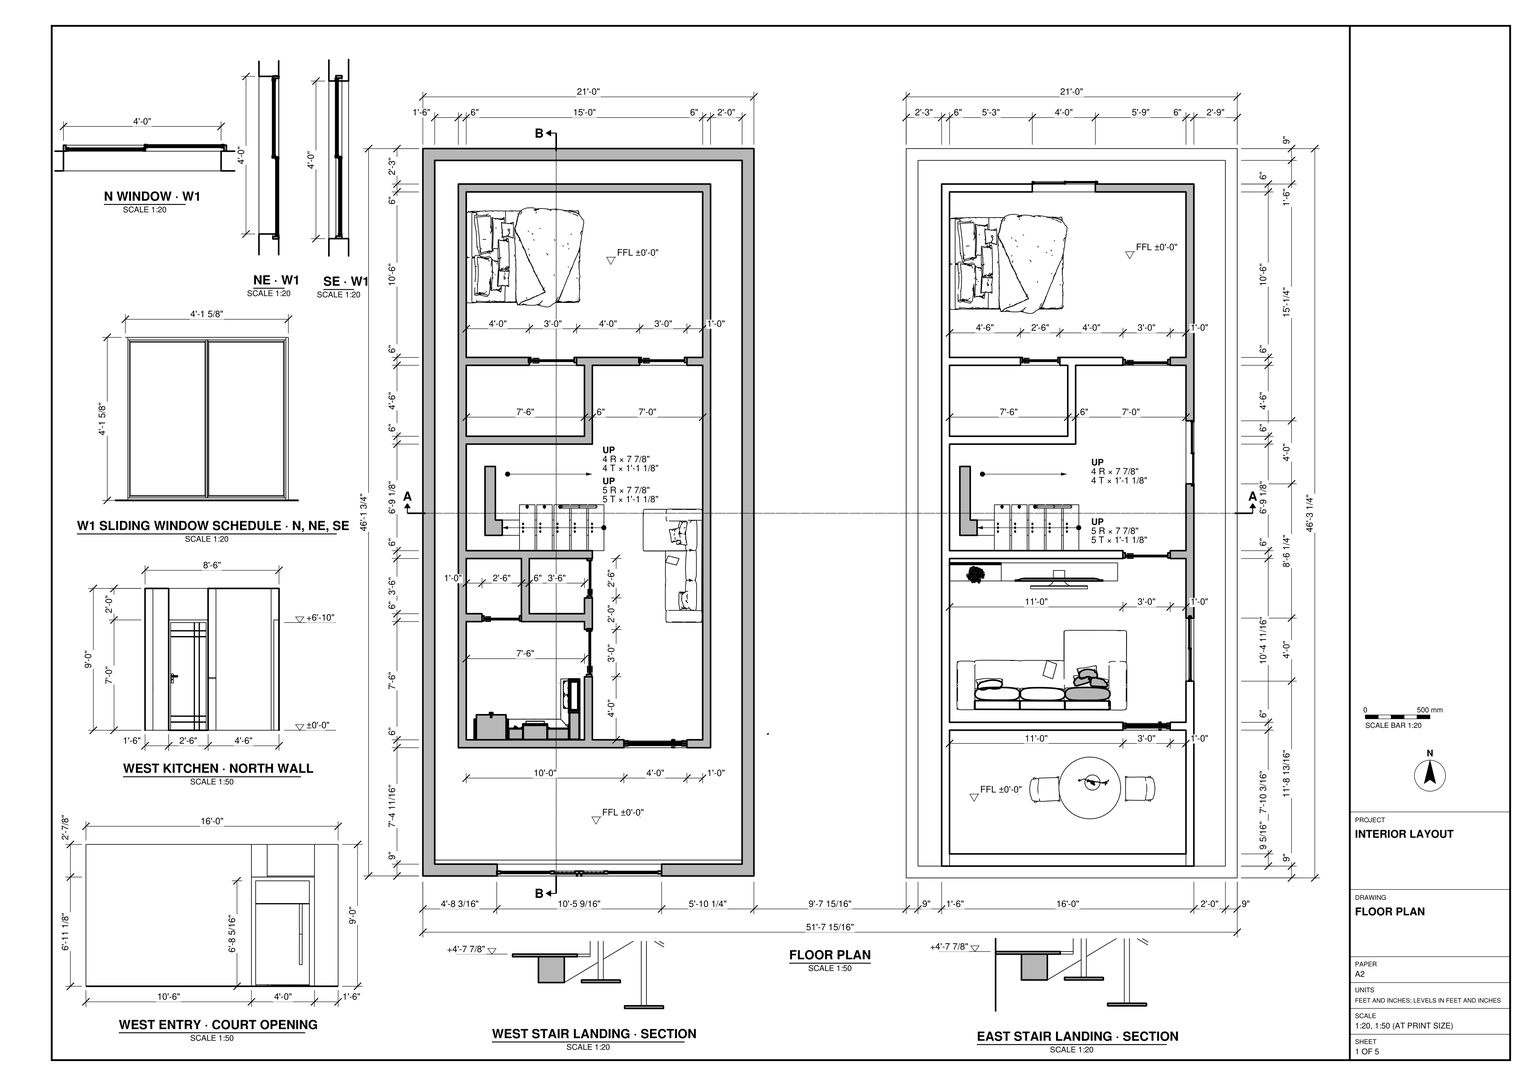
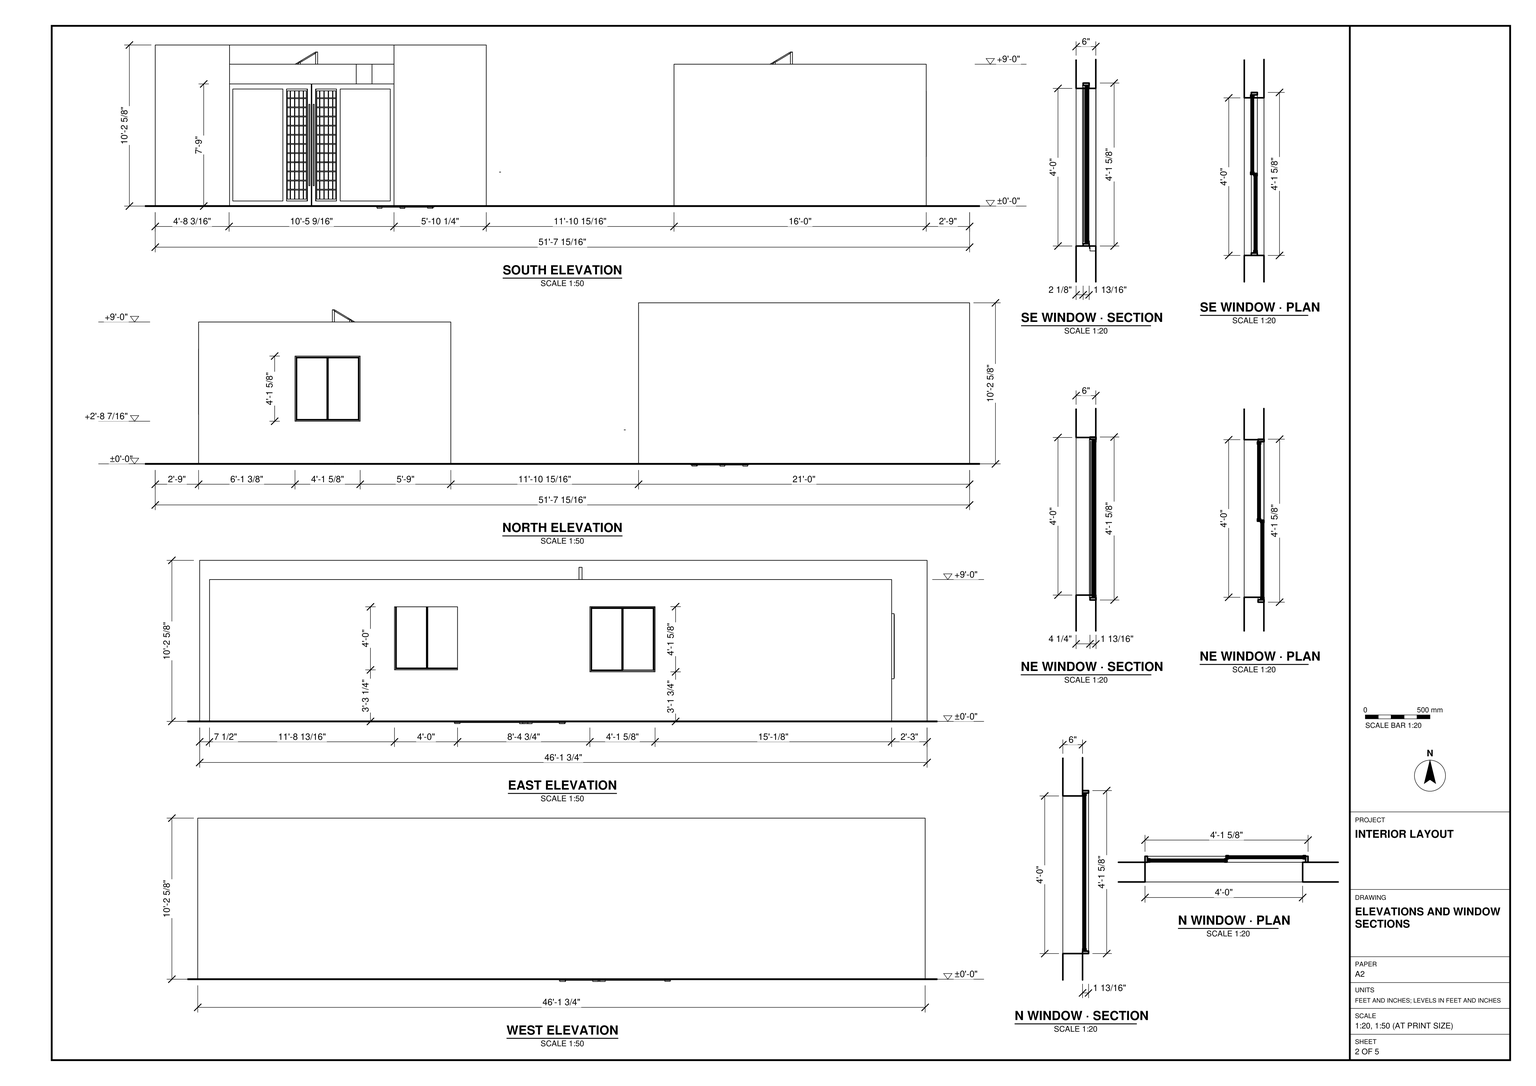
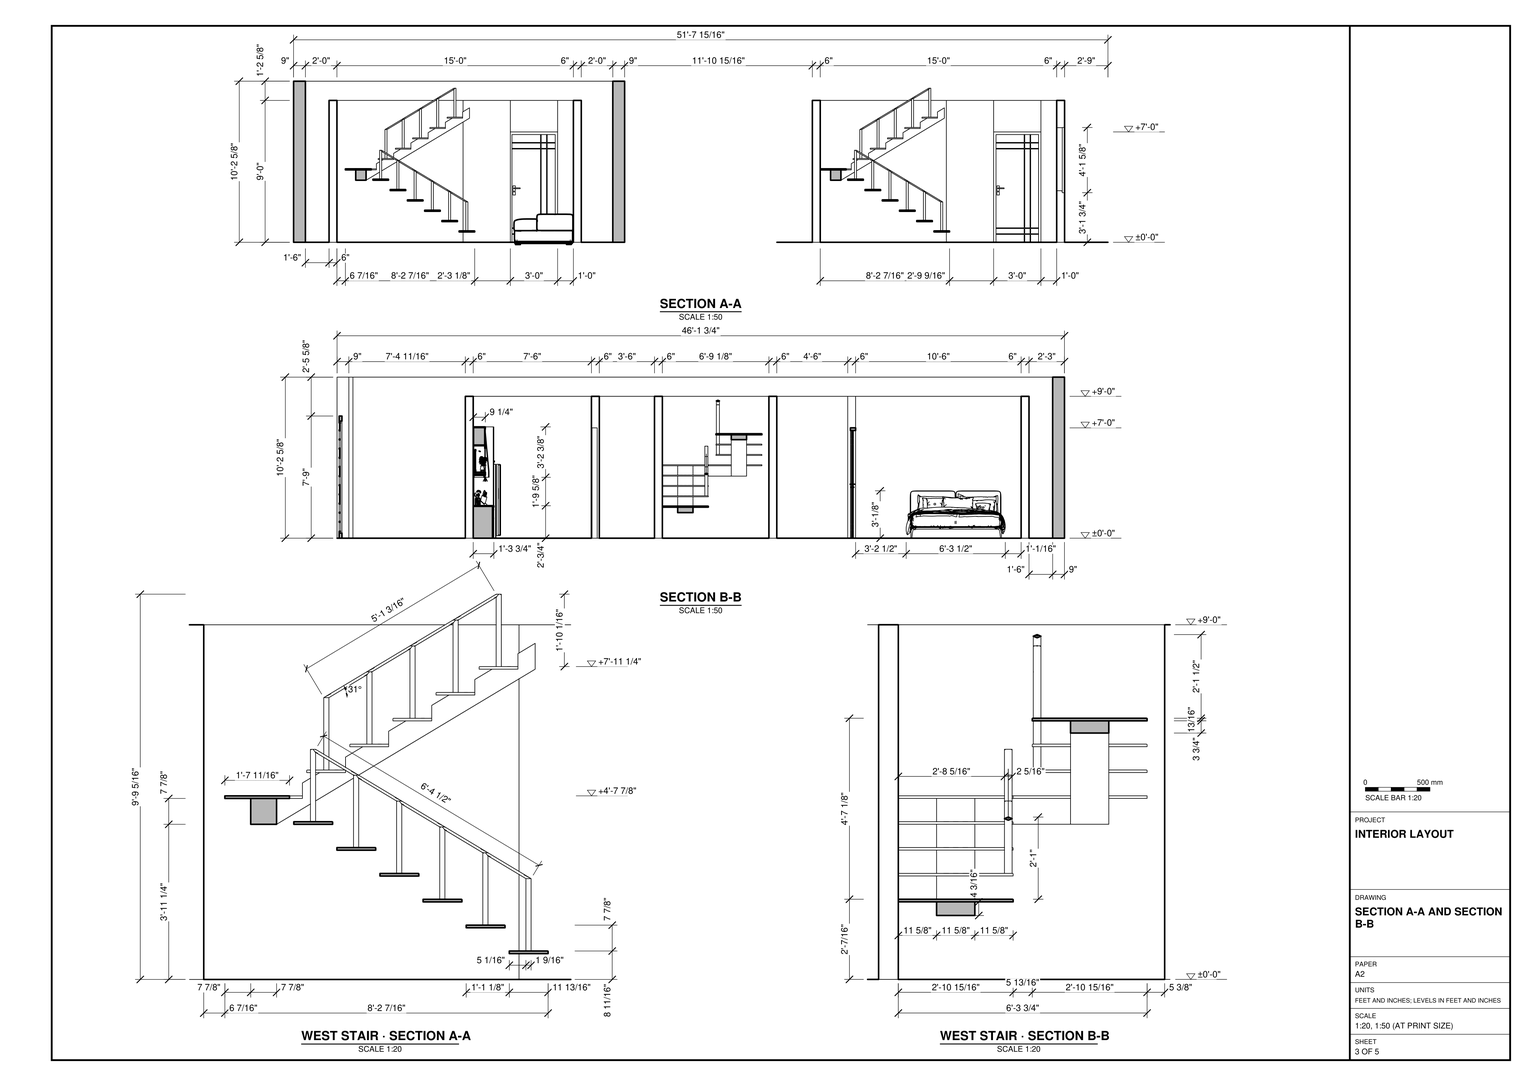
Build both side-by-side layouts in SketchUp from task_files/diagram_01.pdf. Work in feet and inches. Set the finished floor level to ±0'-0" in both layouts. The complete model shall measure 51'-7 15/16" east to west, 46'-3 1/4" north to south and 10'-4 3/8" high. Keep the long axes parallel and use the floor plan to set the gap between the layouts.

Model the floor slabs, the 6" room walls and the taller 9" perimeter walls around the west layout. Form the gated opening into the west entry court and the separate opening from the court into the interior. Place the doors and sliding window units according to the plan, elevations and window details. In the middle of each layout, build the returning stair with individual treads, an intermediate landing, posts and sloping handrails. Use the stair sections to set the heights and the direction in which each flight rises.

Place a bed in each north bedroom. Fit the west kitchen with its L-shaped counter and cabinetry, and place the sofa along the east wall of the west layout. In the east layout, arrange the living room sofa opposite the media unit and furnish the room to its south with the round table and chairs. Match the main furniture and joinery footprints to the plan. Decor, appliances and other loose items may be any suitable library components.

Keep the shell elements and each piece of furniture or joinery in separate groups or components, and use components for repeated parts. Save one SketchUp model as output_files/paired_residential_interiors_and_west_entry_court.skp.

# SketchUp Ruby script. Lengths in inches.
U = 1.inch
M = Sketchup.active_model
def pt(a) = Geom::Point3d.new(a.map { |v| v * U })
def face(e, loops, mat)
  f = e.add_face(loops[0].map { |a| pt(a) })
  loops[1..].each { |l| e.add_face(l.map { |a| pt(a) }).erase! }
  f.material = f.back_material = mat if mat
  f
end
# faces: each face lists its corners as indices into pts; further lists are holes
def faces(e, pts, list, mat = nil) = list.each { |f| face(e, (f[0].is_a?(Array) ? f : [f]).map { |l| l.map { |i| pts[i] } }, mat) }
# xy, xz, yz: faces in a plane at the given z, y or x. An outline is a flat list of corners, or four numbers for a rectangle; further outlines are holes
def ring(l) = l.size == 4 ? [[l[0], l[1]], [l[2], l[1]], [l[2], l[3]], [l[0], l[3]]] : l.each_slice(2).to_a
def flat(e, list, mat, &to3) = list.each { |f| face(e, (f[0].is_a?(Array) ? f : [f]).map { |l| ring(l).map { |u, v| to3.(u, v) } }, mat) }
def xy(e, z, list, mat = nil) = flat(e, list, mat) { |x, y| [x, y, z] }
def xz(e, y, list, mat = nil) = flat(e, list, mat) { |x, z| [x, y, z] }
def yz(e, x, list, mat = nil) = flat(e, list, mat) { |y, z| [x, y, z] }
def lines(e, pts, list) = list.each { |a, b| e.add_line(pt(pts[a]), pt(pts[b])) }
# prism: a flat outline (further loops are holes) pulled along v
def prism(e, loops, v, mat = nil)
  f = face(e, loops, mat); d = Geom::Vector3d.new(v.map { |x| x * U })
  f.pushpull(f.normal.samedirection?(d) ? d.length : -d.length)
end
def box(e, o, s, mat = nil) = prism(e, [[o, [o[0] + s[0], o[1], o[2]], [o[0] + s[0], o[1] + s[1], o[2]], [o[0], o[1] + s[1], o[2]]]], [0, 0, s[2]], mat)
def at(x, y, z, deg = 0) = Geom::Transformation.translation(pt([x, y, z])) * Geom::Transformation.rotation(ORIGIN, Z_AXIS, deg.degrees)
def axes(o, x, y, z) = Geom::Transformation.new([*x, 0, *y, 0, *z, 0, *pt(o).to_a, 1])
def part(name) = M.definitions.add(name)
# library, detail: a bought-in or finely detailed component or shape, given as its bounding box
def library(name, o, s) = part(name).tap { |d| box(d.entities, o, s) }
def detail(e, o, s) = box(e.add_group.entities, o, s)
def put(e, d, t, mat = nil) = e.add_instance(d, t).tap { |i| i.material = mat if mat }
def group(e, t, mat = nil) = e.add_group.tap { |g| g.transformation = t; g.material = mat if mat }.entities
root = M.entities
M.materials.add("Glass_Tinted_Gray").color = [0, 0, 0]
M.materials["Glass_Tinted_Gray"].alpha = 0.125
M.materials.add("[0131_Silver]").color = [192, 192, 192]
M.materials.add("[0135_DarkGray]2").color = [81, 81, 81]
M.materials.add("[Basic Tile]").color = [203, 206, 202]
M.materials.add("[Color M03]").color = [170, 170, 170]
M.materials.add("[Color M05]1").color = [114, 114, 114]
M.materials.add("[Concrete Tile]").color = [203, 190, 164]
M.materials.add("[Field Square Tile]").color = [217, 201, 169]
M.materials.add("[Granite Tile]").color = [155, 148, 143]
M.materials.add("[Grass Dark Green]").color = [106, 157, 55]
M.materials.add("[Metal Panel]").color = [143, 157, 158]
M.materials.add("[Metal_Aluminum_Anodized]").color = [200, 209, 218]
M.materials.add("[Metal_Aluminum_Anodized]1").color = [54, 58, 61]
M.materials.add("[Mirror 02]").color = [229, 229, 229]
M.materials.add("[Quartz Light Brown]").color = [199, 184, 152]
M.materials.add("[Terrazzo Light Blue]").color = [196, 214, 227]
M.materials.add("[Wood Floor]").color = [155, 105, 61]
M.materials.add("[Wood_Board_Cork]").color = [190, 124, 73]
c1 = library("Untitled",[-25.65,-58.99,0],[75.48,89.46,37.24])
c2 = part("porta+1")
xy(c2.entities,21.32,[[44.39,-2.88,46.83,-2.61]],"[Wood_Board_Cork]")
xz(c2.entities,-4.82,[[44.39,41.04,46.83,44.9375]],"[Wood_Board_Cork]")
xz(c2.entities,-4.55,[[44.39,41.05,46.83,44.93]],"[Wood_Board_Cork]")
yz(c2.entities,3.7,[[-2.78,1.36,-3.92,84.5,-2.04,84.53,-0.9,1.39]],"[Wood_Board_Cork]")
yz(c2.entities,7.31,[[-2.79,2.49,-2.35,2.5,-3.4375,81.66,-3.875,81.65]],"[Wood_Board_Cork]")
yz(c2.entities,7.67,[[-2.78,1.36,-0.9,1.39,-0.92,2.51,-2.35,2.5,-2.79,2.49]],"[Wood_Board_Cork]")
yz(c2.entities,9.8,[[-1.42,2.51,-0.92,2.51,-1.99,80.51,-2.49,80.5]],"[Wood_Board_Cork]")
yz(c2.entities,44.39,[[-2.5625,17.82,-3.21,21.66,-3.74,25.52,-4.17,29.39,-4.5,33.26,-4.71,37.15,-4.82,41.04,-4.82,44.9375,-4.71,48.83,-4.49,52.71,-4.17,56.59,-3.74,60.46,-3.2,64.32,-3.15,60.82,-3.42,60.8125,-3.47,60.43,-3.9,56.57,-4.23,52.7,-4.44,48.82,-4.55,44.93,-4.55,41.05,-4.45,37.16,-4.23,33.28,-3.91,29.41,-3.48,25.55,-2.94,21.7,-2.88,21.32,-2.61,21.32]],"[Wood_Board_Cork]")
yz(c2.entities,46.83,[[-2.5625,17.82,-2.61,21.32,-2.88,21.32,-2.94,21.7,-3.48,25.55,-3.91,29.41,-4.23,33.28,-4.45,37.16,-4.55,41.05,-4.55,44.93,-4.44,48.82,-4.23,52.7,-3.9,56.57,-3.47,60.43,-3.42,60.8125,-3.15,60.82,-3.2,64.32,-3.74,60.46,-4.17,56.59,-4.49,52.71,-4.71,48.83,-4.82,44.9375,-4.82,41.04,-4.71,37.15,-4.5,33.26,-4.17,29.39,-3.74,25.52,-3.21,21.66]],"[Wood_Board_Cork]")
yz(c2.entities,52.86,[[-2.78,1.36,-2.79,2.49,-2.35,2.5,-1.42,2.51,-0.92,2.51,-0.9,1.39],[-2.79,2.49,-3.875,81.65,-3.4375,81.66,-2.35,2.5],[-1.42,2.51,-2.49,80.5,-1.99,80.51,-0.92,2.51]],"[Wood_Board_Cork]")
yz(c2.entities,57.25,[[-2.78,1.36,-0.9,1.39,-2.04,84.53,-3.92,84.5]],"[Wood_Board_Cork]")
p = [[7.67,-2.78,1.36],[7.67,-2.79,2.49],[7.31,-2.79,2.49],[7.31,-3.875,81.65],[52.86,-3.875,81.65],[52.86,-2.79,2.49],
  [52.86,-2.78,1.36],[57.25,-2.78,1.36],[57.25,-3.92,84.5],[3.7,-3.92,84.5],[3.7,-2.78,1.36],[3.7,-0.9,1.39],
  [7.67,-0.9,1.39],[52.86,-0.9,1.39],[57.25,-0.9,1.39],[52.86,-0.92,2.51],[52.86,-1.99,80.51],[9.8,-1.99,80.51],
  [9.8,-0.92,2.51],[7.67,-0.92,2.51],[3.7,-2.04,84.53],[57.25,-2.04,84.53],[7.67,-2.35,2.5],[52.86,-2.35,2.5],
  [52.86,-3.4375,81.66],[7.31,-3.4375,81.66],[7.31,-2.35,2.5],[44.39,-3.15,60.82],[44.39,-3.2,64.32],[46.83,-3.2,64.32],
  [46.83,-3.15,60.82],[46.83,-2.61,21.32],[46.83,-2.5625,17.82],[44.39,-2.5625,17.82],[44.39,-2.61,21.32],[52.86,-1.42,2.51],
  [9.8,-1.42,2.51],[9.8,-2.49,80.5],[52.86,-2.49,80.5],[46.83,-3.21,21.66],[44.39,-3.21,21.66],[46.83,-2.94,21.7],
  [46.83,-2.88,21.32],[44.39,-2.88,21.32],[44.39,-2.94,21.7],[46.83,-3.74,25.52],[44.39,-3.74,25.52],[46.83,-3.48,25.55],
  [44.39,-3.48,25.55],[46.83,-4.17,29.39],[44.39,-4.17,29.39],[46.83,-3.91,29.41],[44.39,-3.91,29.41],[46.83,-4.5,33.26],
  [44.39,-4.5,33.26],[46.83,-4.23,33.28],[44.39,-4.23,33.28],[46.83,-4.71,37.15],[44.39,-4.71,37.15],[46.83,-4.45,37.16],
  [44.39,-4.45,37.16],[46.83,-4.82,41.04],[44.39,-4.82,41.04],[46.83,-4.55,41.05],[44.39,-4.55,41.05],[46.83,-4.82,44.9375],
  [46.83,-4.71,48.83],[44.39,-4.71,48.83],[44.39,-4.82,44.9375],[46.83,-4.44,48.82],[46.83,-4.55,44.93],[44.39,-4.55,44.93],
  [44.39,-4.44,48.82],[46.83,-4.49,52.71],[44.39,-4.49,52.71],[46.83,-4.23,52.7],[44.39,-4.23,52.7],[46.83,-4.17,56.59],
  [44.39,-4.17,56.59],[46.83,-3.9,56.57],[44.39,-3.9,56.57],[46.83,-3.74,60.46],[44.39,-3.74,60.46],[46.83,-3.47,60.43],
  [44.39,-3.47,60.43],[46.83,-3.42,60.8125],[44.39,-3.42,60.8125]]
faces(c2.entities,p,[[0,1,2,3,4,5,6,7,8,9,10],[11,12,0,10],[6,13,14,7],[13,15,16,17,18,19,12,11,20,21,14],[[22,23,24,25,26],[27,28,29,30,31,32,33,34]],[2,1,22,26],[35,36,37,38],[35,23,22,19,18,36],
  [32,39,40,33],[31,30,27,34],[41,42,43,44],[39,45,46,40],[47,41,44,48],[45,49,50,46],[51,47,48,52],[49,53,54,50],
  [55,51,52,56],[53,57,58,54],[59,55,56,60],[57,61,62,58],[63,59,60,64],[65,66,67,68],[69,70,71,72],[66,73,74,67],
  [75,69,72,76],[73,77,78,74],[79,75,76,80],[77,81,82,78],[83,79,80,84],[85,83,84,86],[81,29,28,82],[85,86,27,30],
  [17,16,38,37],[4,3,25,24],[21,20,9,8]],"[Wood_Board_Cork]")
c3 = part("vvv")
put(c3.entities,c2,at(0,0,0))
c4 = part("porta+1\#1")
xy(c4.entities,21.32,[[44.39,-2.88,46.83,-2.61]],"[Wood_Board_Cork]")
xz(c4.entities,-4.82,[[44.39,41.04,46.83,44.9375]],"[Wood_Board_Cork]")
xz(c4.entities,-4.55,[[44.39,41.05,46.83,44.93]],"[Wood_Board_Cork]")
yz(c4.entities,3.7,[[-2.78,1.36,-3.92,84.5,-2.04,84.53,-0.9,1.39]],"[Wood_Board_Cork]")
yz(c4.entities,7.31,[[-2.79,2.49,-2.35,2.5,-3.4375,81.66,-3.875,81.65]],"[Wood_Board_Cork]")
yz(c4.entities,7.67,[[-2.78,1.36,-0.9,1.39,-0.92,2.51,-2.35,2.5,-2.79,2.49]],"[Wood_Board_Cork]")
yz(c4.entities,9.8,[[-1.42,2.51,-0.92,2.51,-1.99,80.51,-2.49,80.5]],"[Wood_Board_Cork]")
yz(c4.entities,44.39,[[-2.5625,17.82,-3.21,21.66,-3.74,25.52,-4.17,29.39,-4.5,33.26,-4.71,37.15,-4.82,41.04,-4.82,44.9375,-4.71,48.83,-4.49,52.71,-4.17,56.59,-3.74,60.46,-3.2,64.32,-3.15,60.82,-3.42,60.8125,-3.47,60.43,-3.9,56.57,-4.23,52.7,-4.44,48.82,-4.55,44.93,-4.55,41.05,-4.45,37.16,-4.23,33.28,-3.91,29.41,-3.48,25.55,-2.94,21.7,-2.88,21.32,-2.61,21.32]],"[Wood_Board_Cork]")
yz(c4.entities,46.83,[[-2.5625,17.82,-2.61,21.32,-2.88,21.32,-2.94,21.7,-3.48,25.55,-3.91,29.41,-4.23,33.28,-4.45,37.16,-4.55,41.05,-4.55,44.93,-4.44,48.82,-4.23,52.7,-3.9,56.57,-3.47,60.43,-3.42,60.8125,-3.15,60.82,-3.2,64.32,-3.74,60.46,-4.17,56.59,-4.49,52.71,-4.71,48.83,-4.82,44.9375,-4.82,41.04,-4.71,37.15,-4.5,33.26,-4.17,29.39,-3.74,25.52,-3.21,21.66]],"[Wood_Board_Cork]")
yz(c4.entities,52.86,[[-2.78,1.36,-2.79,2.49,-2.35,2.5,-1.42,2.51,-0.92,2.51,-0.9,1.39],[-2.79,2.49,-3.875,81.65,-3.4375,81.66,-2.35,2.5],[-1.42,2.51,-2.49,80.5,-1.99,80.51,-0.92,2.51]],"[Wood_Board_Cork]")
yz(c4.entities,57.25,[[-2.78,1.36,-0.9,1.39,-2.04,84.53,-3.92,84.5]],"[Wood_Board_Cork]")
p = [[7.67,-2.78,1.36],[7.67,-2.79,2.49],[7.31,-2.79,2.49],[7.31,-3.875,81.65],[52.86,-3.875,81.65],[52.86,-2.79,2.49],
  [52.86,-2.78,1.36],[57.25,-2.78,1.36],[57.25,-3.92,84.5],[3.7,-3.92,84.5],[3.7,-2.78,1.36],[3.7,-0.9,1.39],
  [7.67,-0.9,1.39],[52.86,-0.9,1.39],[57.25,-0.9,1.39],[52.86,-0.92,2.51],[52.86,-1.99,80.51],[9.8,-1.99,80.51],
  [9.8,-0.92,2.51],[7.67,-0.92,2.51],[3.7,-2.04,84.53],[57.25,-2.04,84.53],[7.67,-2.35,2.5],[52.86,-2.35,2.5],
  [52.86,-3.4375,81.66],[7.31,-3.4375,81.66],[7.31,-2.35,2.5],[44.39,-3.15,60.82],[44.39,-3.2,64.32],[46.83,-3.2,64.32],
  [46.83,-3.15,60.82],[46.83,-2.61,21.32],[46.83,-2.5625,17.82],[44.39,-2.5625,17.82],[44.39,-2.61,21.32],[52.86,-1.42,2.51],
  [9.8,-1.42,2.51],[9.8,-2.49,80.5],[52.86,-2.49,80.5],[46.83,-3.21,21.66],[44.39,-3.21,21.66],[46.83,-2.94,21.7],
  [46.83,-2.88,21.32],[44.39,-2.88,21.32],[44.39,-2.94,21.7],[46.83,-3.74,25.52],[44.39,-3.74,25.52],[46.83,-3.48,25.55],
  [44.39,-3.48,25.55],[46.83,-4.17,29.39],[44.39,-4.17,29.39],[46.83,-3.91,29.41],[44.39,-3.91,29.41],[46.83,-4.5,33.26],
  [44.39,-4.5,33.26],[46.83,-4.23,33.28],[44.39,-4.23,33.28],[46.83,-4.71,37.15],[44.39,-4.71,37.15],[46.83,-4.45,37.16],
  [44.39,-4.45,37.16],[46.83,-4.82,41.04],[44.39,-4.82,41.04],[46.83,-4.55,41.05],[44.39,-4.55,41.05],[46.83,-4.82,44.9375],
  [46.83,-4.71,48.83],[44.39,-4.71,48.83],[44.39,-4.82,44.9375],[46.83,-4.44,48.82],[46.83,-4.55,44.93],[44.39,-4.55,44.93],
  [44.39,-4.44,48.82],[46.83,-4.49,52.71],[44.39,-4.49,52.71],[46.83,-4.23,52.7],[44.39,-4.23,52.7],[46.83,-4.17,56.59],
  [44.39,-4.17,56.59],[46.83,-3.9,56.57],[44.39,-3.9,56.57],[46.83,-3.74,60.46],[44.39,-3.74,60.46],[46.83,-3.47,60.43],
  [44.39,-3.47,60.43],[46.83,-3.42,60.8125],[44.39,-3.42,60.8125]]
faces(c4.entities,p,[[0,1,2,3,4,5,6,7,8,9,10],[11,12,0,10],[6,13,14,7],[13,15,16,17,18,19,12,11,20,21,14],[[22,23,24,25,26],[27,28,29,30,31,32,33,34]],[2,1,22,26],[35,36,37,38],[35,23,22,19,18,36],
  [32,39,40,33],[31,30,27,34],[41,42,43,44],[39,45,46,40],[47,41,44,48],[45,49,50,46],[51,47,48,52],[49,53,54,50],
  [55,51,52,56],[53,57,58,54],[59,55,56,60],[57,61,62,58],[63,59,60,64],[65,66,67,68],[69,70,71,72],[66,73,74,67],
  [75,69,72,76],[73,77,78,74],[79,75,76,80],[77,81,82,78],[83,79,80,84],[85,83,84,86],[81,29,28,82],[85,86,27,30],
  [17,16,38,37],[4,3,25,24],[21,20,9,8]],"[Wood_Board_Cork]")
put(c4.entities,c3,axes([0,-1.9375,-0.02],[1,0,0],[0,-0.99945,-0.03316],[0,-0.03316,0.99945]))
c5 = part("porta+de+madeira")
prism(c5.entities,[[[7.31,-2.51,64.03],[52.86,-2.51,64.03],[52.86,-3.01,64.03],[7.31,-3.01,64.03]]],[0,-0.01,0.4])
put(c5.entities,c4,at(0,0,0))
c6 = library("Untitled (1)",[0,0,0],[36,4.39,84])
c7 = library("Sectional sofa",[-0.93,-10.63,-23.92],[126.92,88.46,78.25])
c8 = part("Agrupar\#1")
xy(c8.entities,0,[[0,0,0,2.36,13.27,2.36,13.6875,2.5,14.09,2.66,14.48,2.84,14.86,3.05,15.23,3.28,15.59,3.54,15.92,3.8125,16.24,4.11,16.54,4.42,16.82,4.75,17.08,5.1,17.32,5.46,17.32,13.99,25.98,13.99,25.98,5.46,26.22,5.1,26.48,4.74,26.76,4.41,27.06,4.1,27.375,3.8,27.71,3.52,28.07,3.27,28.43,3.04,28.82,2.83,29.21,2.65,29.62,2.49,30.03,2.36,43.31,2.36,43.31,0]],"[Metal_Aluminum_Anodized]1")
xy(c8.entities,0.59,[[0,1.97,43.31,2.36],[13.27,2.36,30.03,2.36,29.62,2.49,29.21,2.65,28.82,2.83,28.43,3.04,28.07,3.27,27.71,3.52,27.375,3.8,27.06,4.1,26.76,4.41,26.48,4.74,26.22,5.1,25.98,5.46,25.98,12.02,17.32,12.02,17.32,5.46,17.08,5.1,16.82,4.75,16.54,4.42,16.24,4.11,15.92,3.8125,15.59,3.54,15.23,3.28,14.86,3.05,14.48,2.84,14.09,2.66,13.6875,2.5]],"[Metal_Aluminum_Anodized]1")
xz(c8.entities,0,[[0,0,43.31,0.2]],"[Metal_Aluminum_Anodized]1")
xz(c8.entities,2.36,[[0,0,13.27,0.59],[30.03,0,43.31,0.59]],"[Metal_Aluminum_Anodized]1")
xz(c8.entities,8.32,[[17.32,4.9375,25.98,7.25]],"[Metal_Aluminum_Anodized]1")
xz(c8.entities,13.99,[[17.32,0,25.98,0.59]],"[Metal_Aluminum_Anodized]1")
yz(c8.entities,0,[[0,0,0,0.2,1.97,0.59,1.97,0],[1.97,0,2.36,0.59]],"[Metal_Aluminum_Anodized]1")
yz(c8.entities,17.32,[[5.46,0,5.46,0.59,12.02,0.59,8.32,4.9375,8.32,7.25,13.99,0.59,13.99,0]],"[Metal_Aluminum_Anodized]1")
yz(c8.entities,25.98,[[5.46,0,13.99,0,13.99,0.59,8.32,7.25,8.32,4.9375,12.02,0.59,5.46,0.59]],"[Metal_Aluminum_Anodized]1")
yz(c8.entities,43.31,[[0,0,1.97,0,1.97,0.59,0,0.2],[1.97,0,2.36,0.59]],"[Metal_Aluminum_Anodized]1")
p = [[13.6875,2.5,0],[13.27,2.36,0],[13.27,2.36,0.59],[13.6875,2.5,0.59],[30.03,2.36,0],[29.62,2.49,0],
  [29.62,2.49,0.59],[30.03,2.36,0.59],[14.09,2.66,0],[14.09,2.66,0.59],[29.21,2.65,0],[29.21,2.65,0.59],
  [14.48,2.84,0],[14.48,2.84,0.59],[28.82,2.83,0],[28.82,2.83,0.59],[14.86,3.05,0],[14.86,3.05,0.59],
  [28.43,3.04,0],[28.43,3.04,0.59],[28.07,3.27,0],[28.07,3.27,0.59],[15.23,3.28,0],[15.23,3.28,0.59],
  [15.59,3.54,0],[15.59,3.54,0.59],[27.71,3.52,0],[27.71,3.52,0.59],[15.92,3.8125,0],[15.92,3.8125,0.59],
  [27.375,3.8,0],[27.375,3.8,0.59],[16.24,4.11,0],[16.24,4.11,0.59],[27.06,4.1,0],[27.06,4.1,0.59],
  [16.54,4.42,0],[16.54,4.42,0.59],[26.76,4.41,0],[26.76,4.41,0.59],[16.82,4.75,0],[16.82,4.75,0.59],
  [26.48,4.74,0],[26.48,4.74,0.59],[26.22,5.1,0],[26.22,5.1,0.59],[17.08,5.1,0],[17.08,5.1,0.59],
  [17.32,5.46,0],[17.32,5.46,0.59],[25.98,5.46,0],[25.98,5.46,0.59],[43.31,0,0.2],[43.31,1.97,0.59],
  [0,1.97,0.59],[0,0,0.2],[25.98,13.99,0.59],[25.98,8.32,7.25],[17.32,8.32,7.25],[17.32,13.99,0.59],
  [25.98,8.32,4.9375],[25.98,12.02,0.59],[17.32,12.02,0.59],[17.32,8.32,4.9375]]
faces(c8.entities,p,[[0,1,2,3],[4,5,6,7],[8,0,3,9],[5,10,11,6],[12,8,9,13],[10,14,15,11],[16,12,13,17],[14,18,19,15],
  [18,20,21,19],[22,16,17,23],[24,22,23,25],[20,26,27,21],[28,24,25,29],[26,30,31,27],[32,28,29,33],[30,34,35,31],
  [36,32,33,37],[34,38,39,35],[40,36,37,41],[38,42,43,39],[42,44,45,43],[46,40,41,47],[48,46,47,49],[44,50,51,45],
  [56,57,58,59],[60,61,62,63]],"[Metal_Aluminum_Anodized]1")
faces(c8.entities,p,[[52,53,54,55]],"[Metal_Aluminum_Anodized]")
c9 = library("Agrupar\#2",[0,0,0],[66.49,2.6,38.28])
c10 = part("Samsung 75")
p = [[0,0,0],[1,0,0],[1,1,0]]
lines(c10.entities,p,[[0,1],[1,2],[2,0]])
put(c10.entities,c8,at(200.625,110.82,-2.44),"[Metal_Aluminum_Anodized]")
put(c10.entities,c9,at(189.03,116.54,0))
c11 = library("Vtufgjkbc",[-37.34,-38.3,0],[76.68,71.13,141.17])
c12 = part("Enscape.LinearLight")
xz(c12.entities,-44.64,[[0,-1,0,0,-0.38,-0.92],[0,-1,0.38,-0.92,0,0],[-0.38,-0.92,0,0,-0.71,-0.71],[0.38,-0.92,0.71,-0.71,0,0],[-0.71,-0.71,0,0,-0.92,-0.38],
  [0.71,-0.71,0.92,-0.38,0,0],[-0.92,-0.38,0,0,-1,0],[0.92,-0.38,1,0,0,0],[-1,0,0,0,-0.92,0.38],[0,0,-0.71,0.71,-0.92,0.38],
  [0,0,-0.38,0.92,-0.71,0.71],[0,0,0,1,-0.38,0.92],[0,0,0.38,0.92,0,1],[0,0,0.71,0.71,0.38,0.92],[0,0,0.92,0.38,0.71,0.71],
  [0,0,1,0,0.92,0.38]])
xz(c12.entities,44.64,[[0,-1,-0.38,-0.92,0,0],[0,-1,0,0,0.38,-0.92],[-0.38,-0.92,-0.71,-0.71,0,0],[0.38,-0.92,0,0,0.71,-0.71],[-0.71,-0.71,-0.92,-0.38,0,0],
  [0.71,-0.71,0,0,0.92,-0.38],[-0.92,-0.38,-1,0,0,0],[0.92,-0.38,0,0,1,0],[-1,0,-0.92,0.38,0,0],[0,0,-0.92,0.38,-0.71,0.71],
  [0,0,-0.71,0.71,-0.38,0.92],[0,0,-0.38,0.92,0,1],[0,0,0,1,0.38,0.92],[0,0,0.38,0.92,0.71,0.71],[0,0,0.71,0.71,0.92,0.38],
  [0,0,0.92,0.38,1,0]])
p = [[-0.38,-44.64,-0.92],[-0.38,44.64,-0.92],[0,44.64,-1],[0,-44.64,-1],[0.38,44.64,-0.92],[0.38,-44.64,-0.92],
  [-0.71,-44.64,-0.71],[-0.71,44.64,-0.71],[0.71,44.64,-0.71],[0.71,-44.64,-0.71],[-0.92,-44.64,-0.38],[-0.92,44.64,-0.38],
  [0.92,44.64,-0.38],[0.92,-44.64,-0.38],[-1,-44.64,0],[-1,44.64,0],[1,44.64,0],[1,-44.64,0],
  [-0.92,-44.64,0.38],[-0.92,44.64,0.38],[0.92,44.64,0.38],[0.92,-44.64,0.38],[-0.71,-44.64,0.71],[-0.71,44.64,0.71],
  [0.71,44.64,0.71],[0.71,-44.64,0.71],[-0.38,-44.64,0.92],[-0.38,44.64,0.92],[0.38,44.64,0.92],[0.38,-44.64,0.92],
  [0,-44.64,1],[0,44.64,1]]
faces(c12.entities,p,[[0,1,2],[0,2,3],[3,2,4],[3,4,5],[6,7,1],[6,1,0],[5,4,8],[5,8,9],
  [10,11,7],[10,7,6],[9,8,12],[9,12,13],[14,15,11],[14,11,10],[13,12,16],[13,16,17],
  [18,19,15],[18,15,14],[17,16,20],[17,20,21],[22,23,19],[22,19,18],[21,20,24],[21,24,25],
  [26,27,23],[26,23,22],[25,24,28],[25,28,29],[30,31,27],[30,27,26],[29,28,31],[29,31,30]])
c13 = part("Group\#4")
box(c13.entities,[0,0,0],[1.57,1.18,81.22])
c14 = part("tv unit")
put(c14.entities,c10,at(-134.98,-45.95,38.54))
put(c14.entities,c11,axes([23.51,76.07,18.38],[0.185,0,0],[0,0.185,0],[0,0,0.185]))
put(c14.entities,c12,axes([87.75,81.2,82.67],[-0.0192,0.99911,-0.03748],[-0.99982,-0.01919,0.00072],[0,0.03749,0.9993]))
g1 = group(c14.entities,at(3.9375,84.65,12.68))
box(g1,[0,-13.78,0],[127.95,13.78,5.79])
g2 = group(c14.entities,at(43.31,84.65,18.46))
prism(g2,[[[0,0,0],[88.58,0,0],[88.58,-13.78,0],[59.21,-13.78,0],[59.21,-12.99,0],[59.06,-12.99,0],[59.06,-13.78,0],[29.69,-13.78,0],[29.69,-12.99,0],[29.53,-12.99,0],[29.53,-13.78,0],[0,-13.78,0]]],[0,0,12.6])
g3 = group(c14.entities,at(3.9375,84.65,18.46))
put(g3,c13,at(0,-1.18,0))
g4 = group(g3,at(1.97,-1.18,0))
box(g4,[0,0,0],[1.57,1.18,81.22])
put(g3,c13,at(3.9375,-1.18,0))
put(g3,c13,at(5.91,-1.18,0))
g5 = group(g3,at(7.875,-1.18,0))
box(g5,[0,0,0],[1.57,1.18,81.22])
put(g3,c13,at(9.84,-1.18,0))
put(g3,c13,at(11.8125,-1.18,0))
put(g3,c13,at(13.78,-1.18,0))
put(g3,c13,at(15.75,-1.18,0))
put(g3,c13,at(17.72,-1.18,0))
put(g3,c13,at(19.69,-1.18,0))
put(g3,c13,at(21.65,-1.18,0))
put(g3,c13,at(23.62,-1.18,0))
g6 = group(g3,at(25.59,-1.18,0))
box(g6,[0,0,0],[1.57,1.18,81.22])
put(g3,c13,at(27.56,-1.18,0))
put(g3,c13,at(29.53,-1.18,0))
put(g3,c13,at(31.5,-1.18,0))
put(g3,c13,at(33.46,-1.18,0))
put(g3,c13,at(35.43,-1.18,0))
put(g3,c13,at(37.4,-1.18,0))
g7 = group(c14.entities,at(42.91,84.65,81.97))
box(g7,[0,-11.8125,0],[88.98,11.8125,1.97])
c15 = part("PENTEK_RP Fineline 50S_Sliding_DoorCase_E1")
box(c15.entities,[0,0,0],[1.51,3.66,99.27],"[0135_DarkGray]2")
c16 = part("PENTEK_RP Fineline 50S_SlidingDooe_Case_E2")
box(c16.entities,[0,0,0],[96.25,3.66,1.51],"[0135_DarkGray]2")
c17 = part("pentek_RP Fineline 50S_SlidingDoor_Case")
put(c17.entities,c15,at(97.76,0,0))
put(c17.entities,c16,at(1.51,0,0))
put(c17.entities,c15,at(0,0,0))
put(c17.entities,c16,at(1.51,0,97.76))
c18 = part("PENTEK_RP Fineline 50S_SlidingDoor_GlazingBead_2")
box(c18.entities,[0,0,0],[0.56,0.59,94.39],"[0135_DarkGray]2")
c19 = part("PENTEK_RP Fineline 50S_SlidingDoor_Glass")
box(c19.entities,[0,0,0],[46.58,0.16,94.39],"Glass_Tinted_Gray")
c20 = part("PENTEK_RP Fineline 50S_SlidingDoor_GlazingBead")
box(c20.entities,[0,0,0],[45.47,0.59,0.56],"[0135_DarkGray]2")
c21 = part("PENTEK_RP Fineline 50S_SlidingDoor_Leaf_E1")
xy(c21.entities,0,[[0,0,0.93,1.97],[0.93,1.57,1.49,1.97]],"[0135_DarkGray]2")
xy(c21.entities,96.25,[[0,0,0.93,0,0.93,1.57,1.49,1.57,1.49,1.97,0,1.97]],"[0135_DarkGray]2")
xz(c21.entities,0,[[0,0,0.93,96.25]],"[0135_DarkGray]2")
xz(c21.entities,1.57,[[0.93,0,1.49,95.32],[0.93,95.32,1.49,96.25]],"[0135_DarkGray]2")
xz(c21.entities,1.97,[[0,0,1.49,96.25]],"[0135_DarkGray]2")
yz(c21.entities,0,[[0,0,1.97,96.25]],"[0135_DarkGray]2")
yz(c21.entities,0.93,[[0,0,1.57,0.93],[0,0.93,1.57,95.32],[0,95.32,1.57,96.25]],"[0135_DarkGray]2")
yz(c21.entities,1.49,[[1.57,0,1.97,95.32],[1.57,95.32,1.97,96.25]],"[0135_DarkGray]2")
c22 = part("PENTEK_RP Fineline 50S_SlidingDoor_Leaf_E2")
xy(c22.entities,0,[[0,0,0,1.57,0.56,1.57,0.56,1.97,46.02,1.97,46.02,1.57,46.58,1.57,46.58,0]],"[0135_DarkGray]2")
xy(c22.entities,0.93,[[0,0,46.58,1.57]],"[0135_DarkGray]2")
xy(c22.entities,1.49,[[0.56,1.57,46.02,1.97]],"[0135_DarkGray]2")
xz(c22.entities,0,[[0,0,46.58,0.93]],"[0135_DarkGray]2")
xz(c22.entities,1.57,[[0,0,0.56,0.93],[46.02,0,46.58,0.93],[0.56,0.93,46.02,1.49]],"[0135_DarkGray]2")
xz(c22.entities,1.97,[[0.56,0,46.02,1.49]],"[0135_DarkGray]2")
yz(c22.entities,0,[[0,0,1.57,0.93]],"[0135_DarkGray]2")
yz(c22.entities,0.56,[[1.57,0,1.97,0.93],[1.57,0.93,1.97,1.49]],"[0135_DarkGray]2")
yz(c22.entities,46.02,[[1.57,0,1.97,0.93],[1.57,0.93,1.97,1.49]],"[0135_DarkGray]2")
yz(c22.entities,46.58,[[0,0,1.57,0.93]],"[0135_DarkGray]2")
c23 = part("PENTEK_RP Fineline S_SlidingDoor_Leaf1")
put(c23.entities,c18,at(0.93,0,0.93))
put(c23.entities,c18,at(46.96,0,0.93))
put(c23.entities,c19,at(1.49,1.42,0.93))
put(c23.entities,c20,at(1.49,0,0.93))
put(c23.entities,c19,at(1.49,0.59,0.93),"[Terrazzo Light Blue]")
put(c23.entities,c21,at(0,0,0))
put(c23.entities,c21,axes([48.44,0,0],[-1,0,0],[0,1,0],[0,0,1]))
put(c23.entities,c22,axes([0.93,0,96.25],[1,0,0],[0,1,0],[0,0,-1]))
put(c23.entities,c22,at(0.93,0,0))
put(c23.entities,c20,at(1.49,0,94.77))
c24 = part("PENTEK_RP Fineline 50S_SlidingDoor_Leaf2")
put(c24.entities,c19,at(1.49,1.42,0.93))
put(c24.entities,c20,at(1.49,0,94.77))
put(c24.entities,c18,at(46.96,0,0.93))
put(c24.entities,c19,at(1.49,0.59,0.93),"[Mirror 02]")
put(c24.entities,c18,at(0.93,0,0.93))
put(c24.entities,c21,at(0,0,0))
put(c24.entities,c21,axes([48.44,0,0],[-1,0,0],[0,1,0],[0,0,1]))
put(c24.entities,c20,at(1.49,0,0.93))
put(c24.entities,c22,axes([0.93,0,96.25],[1,0,0],[0,1,0],[0,0,-1]))
put(c24.entities,c22,at(0.93,0,0))
c25 = part("PENTEK - Slimmest Steel Sliding Door / Window\#1")
put(c25.entities,c17,at(0,-1.88,-0.09))
put(c25.entities,c23,at(1.51,-2.27,1.42))
put(c25.entities,c24,at(49.32,-0.3,1.42))
c26 = library("Stairs",[1.13,22.74,0],[98.43,51.19,117.32])
c27 = library("7 tủ bếp",[0,0,0],[77.01,133.86,108.66])
c28 = library("Group",[-23.5,-23.5,-29.13],[47,47,29.33])
c29 = library("Group1",[-12.79,-7.3125,-5.78],[23,32.7,12.01])
c30 = library("Group7",[-9.42,-22.14,-3.66],[18.84,31.3,22.58])
c31 = part("Component\#26")
prism(c31.entities,[[[0.35,0,3.8],[0.35,0,3],[0.35,-1.5,3],[0.35,-1.5,51],[0.35,0,51],[0.35,0,50.2],[0.35,-1,50.2],[0.35,-1,3.8]]],[0.8,0,0])
c32 = part("Framed panel")
xy(c32.entities,0,[[[0,0,66,72],[3,3,43.23,69],[46.23,3,63,69]]])
xy(c32.entities,0.5,[[3,3,43.23,69]])
xy(c32.entities,1.5,[[3,3,43.23,69]])
xy(c32.entities,2,[[[0,0,66,72],[3,3,43.23,69],[46.23,3,63,69]]])
xz(c32.entities,0,[[0,0,46.23,2],[46.23,0,66,2]])
xz(c32.entities,3,[[3,0,27,0.5],[27,0,43.23,0.5],[46.23,0,63,2],[3,1.5,43.23,2]])
xz(c32.entities,69,[[3,0,43.23,0.5],[46.23,0,63,2],[3,1.5,43.23,2]])
xz(c32.entities,72,[[0,0,66,2]])
yz(c32.entities,0,[[0,0,72,2]])
yz(c32.entities,3,[[3,0,69,0.5],[3,1.5,69,2]])
yz(c32.entities,43.23,[[3,0,69,0.5],[3,1.5,69,2]])
yz(c32.entities,46.23,[[3,0,69,2]])
yz(c32.entities,63,[[3,0,69,2]])
yz(c32.entities,66,[[0,0,72,2]])
c33 = part("Group\#130")
box(c33.entities,[0,0,0],[46,0.5,0.5])
c34 = part("Group\#131")
xy(c34.entities,0,[[0,0,4.1875,8.86]],"[Color M03]")
c35 = part("Group\#134")
xy(c35.entities,0,[[0,0,4.1875,8.86]],"[Color M03]")
c36 = part("Decorative screen panel")
put(c36.entities,c32,axes([0,2,0],[1,0,0],[0,0,1],[0,-1,0]),"[0131_Silver]")
g8 = group(c36.entities,at(79.2,1,54.05),"[Color M05]1")
g9 = group(g8,at(-5.38,0,-49.99))
put(g9,c33,axes([-13.96,0,0],[0,0,1.38854],[-0.68806,0,0],[0,-1,0]))
put(g9,c33,axes([-17.45,0,0],[0,0,1.38854],[-0.68806,0,0],[0,-1,0]))
put(g9,c33,axes([-20.9375,0,0],[0,0,1.38854],[-0.68806,0,0],[0,-1,0]))
put(g9,c33,axes([-24.43,0,0],[0,0,1.38854],[-0.68806,0,0],[0,-1,0]))
g10 = group(g8,at(0,0,0))
xy(g10,-51.05,[[-33.03,-1,-16.51,0]])
xy(g10,-49.99,[[-32.34,-1,-17.2,0]])
xy(g10,13.89,[[-32.34,-1,-17.2,0]])
xy(g10,14.95,[[-33.03,-1,-16.51,0]])
xz(g10,-1,[[[-33.03,-51.05,-16.51,14.95],[-32.34,-49.99,-17.2,13.89]]])
yz(g10,-33.03,[[-1,-51.05,0,14.95]])
yz(g10,-32.34,[[-1,-49.99,0,13.89]])
yz(g10,-17.2,[[-1,-49.99,0,13.89]])
yz(g10,-16.51,[[-1,-51.05,0,14.95]])
g11 = group(g8,at(-0.6875,-0.5,-6.38))
put(g11,c33,axes([-16.51,0,0],[-0.32907,0,0],[0,0,-1.06351],[0,-1,0]))
put(g11,c33,axes([-16.51,0,-5.39],[-0.32907,0,0],[0,0,-1.06351],[0,-1,0]))
put(g11,c33,axes([-16.51,0,-10.79],[-0.32907,0,0],[0,0,-1.06351],[0,-1,0]))
put(g11,c33,axes([-16.51,0,-16.18],[-0.32907,0,0],[0,0,-1.06351],[0,-1,0]))
put(g11,c33,axes([-16.51,0,-21.57],[-0.32907,0,0],[0,0,-1.06351],[0,-1,0]))
put(g11,c33,axes([-16.51,0,-26.97],[-0.32907,0,0],[0,0,-1.06351],[0,-1,0]))
put(g11,c33,axes([-16.51,0,-32.36],[-0.32907,0,0],[0,0,-1.06351],[0,-1,0]))
put(g11,c33,axes([-16.51,0,-37.75],[-0.32907,0,0],[0,0,-1.06351],[0,-1,0]))
put(g11,c33,axes([-16.51,0,5.39],[-0.32907,0,0],[0,0,-1.06351],[0,-1,0]))
put(g11,c33,axes([-16.51,0,10.79],[-0.32907,0,0],[0,0,-1.06351],[0,-1,0]))
put(g11,c33,axes([-16.51,0,16.18],[-0.32907,0,0],[0,0,-1.06351],[0,-1,0]))
put(g8,c34,axes([-23.17,-0.5,-44.67],[-0.75119,0,0],[0,0,-0.6],[0,-1,0]))
put(g8,c34,axes([-26.66,-0.5,-33.42],[-0.75119,0,0],[0,0,-1.2],[0,-1,0]))
put(g8,c34,axes([-23.17,-0.5,-28.03],[-0.75119,0,0],[0,0,-1.2],[0,-1,0]))
put(g8,c35,axes([-23.17,-0.5,-27.96],[0,0,1.16108],[-0.35491,0,0],[0,-1,0]))
put(g8,c35,axes([-17.2,-0.5,-38.74],[0,0,1.16108],[-0.24134,0,0],[0,-1,0]))
put(g8,c35,axes([-19.68,-0.5,-44.14],[0,0,1.16108],[-0.35491,0,0],[0,-1,0]))
put(g8,c35,axes([-19.68,-0.5,-17.17],[0,0,1.16108],[-0.35491,0,0],[0,-1,0]))
put(g8,c35,axes([-26.66,-0.5,-11.77],[0,0,1.16108],[-0.35491,0,0],[0,-1,0]))
put(g8,c35,axes([-30.15,-0.5,-27.96],[0,0,1.16108],[-0.35491,0,0],[0,-1,0]))
put(g8,c35,axes([-19.68,-0.5,-6.38],[0,0,1.16108],[-0.35491,0,0],[0,-1,0]))
put(g8,c35,axes([-23.17,-0.5,-6.38],[0,0,1.16108],[-0.35491,0,0],[0,-1,0]))
put(g8,c35,axes([-26.66,-0.5,-0.99],[0,0,1.16108],[-0.35491,0,0],[0,-1,0]))
put(g8,c35,axes([-23.17,-0.5,4.41],[0,0,1.16108],[-0.35491,0,0],[0,-1,0]))
put(g8,c35,axes([-23.17,-0.5,-17.17],[0,0,1.16108],[-0.35491,0,0],[0,-1,0]))
put(g8,c35,axes([-19.68,-0.5,-33.35],[0,0,1.16108],[-0.35491,0,0],[0,-1,0]))
put(g8,c35,axes([-26.66,-0.5,-22.5625],[0,0,1.16108],[-0.35491,0,0],[0,-1,0]))
put(g8,c35,axes([-19.68,-0.5,9.8],[0,0,1.16108],[-0.35491,0,0],[0,-1,0]))
put(g8,c35,axes([-23.17,-0.5,9.8],[0,0,1.16108],[-0.35491,0,0],[0,-1,0]))
put(g8,c35,axes([-26.66,-0.5,4.41],[0,0,1.16108],[-0.35491,0,0],[0,-1,0]))
put(g8,c35,axes([-19.68,-0.5,-0.99],[0,0,1.16108],[-0.35491,0,0],[0,-1,0]))
put(g8,c34,axes([-26.66,-0.5,-44.67],[-0.75119,0,0],[0,0,-0.6],[0,-1,0]))
g12 = group(g8,at(-16.2,-0.5,-44.67))
xz(g12,0,[[-3.15,-5.32,-1.01,0]],"[Color M03]")
put(g8,c34,axes([-30.17,-0.5,-28.49],[-0.51832,0,0],[0,0,-0.54857],[0,-1,0]))
put(g8,c35,axes([-17.2,-0.5,-27.96],[0,0,1.16108],[-0.24134,0,0],[0,-1,0]))
put(g8,c35,axes([-17.2,-0.5,-22.5625],[0,0,1.16108],[-0.24134,0,0],[0,-1,0]))
put(g8,c35,axes([-17.2,-0.5,-11.77],[0,0,1.16108],[-0.24134,0,0],[0,-1,0]))
put(g8,c35,axes([-17.2,-0.5,4.41],[0,0,1.16108],[-0.24134,0,0],[0,-1,0]))
put(g8,c35,axes([-30.15,-0.5,-17.17],[0,0,1.16108],[-0.35491,0,0],[0,-1,0]))
put(g8,c35,axes([-30.15,-0.5,-6.38],[0,0,1.16108],[-0.35491,0,0],[0,-1,0]))
put(g8,c35,axes([-30.15,-0.5,9.8],[0,0,0.9764],[-0.35491,0,0],[0,-1,0]))
xy(root,0,[[[367.91,0,619.91,555.25],[376.91,9,610.91,546.25]],[0,1.48,0,555.25,252,555.25,252,1.48,181.75,1.48,181.75,10.48,243,10.48,243,546.25,9,546.25,9,10.48,56.5625,10.48,56.5625,1.48],[56.5625,1.48,181.75,10.48],[9,10.48,243,13.58]])
xy(root,0,[[376.91,9,394.91,9,394.91,528.25,586.91,528.25,586.91,9,610.91,9,610.91,546.25,376.91,546.25]],"[Concrete Tile]")
xy(root,0,[[153,99.14,201,99.14,201,105.14,213,105.14,213,390.25,129,390.25,129,330.25,33,330.25,33,249.14,129,249.14,129,243.14,81,243.14,81,201.14,123,201.14,123,213.14,129,213.14,129,189.14,123,189.14,123,195.14,75,195.14,75,243.14,33,243.14,33,201.14,45,201.14,45,195.14,33,195.14,33,105.14,123,105.14,123,153.14,129,153.14,129,105.14,153,105.14],[532.91,112.48,568.91,112.48,568.91,118.48,580.91,118.48,580.91,243.14,568.91,243.14,568.91,249.14,580.91,249.14,580.91,390.25,496.91,390.25,496.91,330.25,400.91,330.25,400.91,249.14,532.91,249.14,532.91,243.14,400.91,243.14,400.91,118.48,532.91,118.48]],"[Field Square Tile]")
xy(root,0,[[[9,13.58,243,546.25],[27,99.14,219,528.25]]],"[Granite Tile]")
xy(root,0,[[400.91,18.29,580.91,112.48]],"[Grass Dark Green]")
xy(root,0,[[33,336.25,123,390.25],[400.91,336.25,490.91,390.25]],"[Metal Panel]")
xy(root,0,[[81,390.25,117,390.25,117,396.25,165,396.25,165,390.25,201,390.25,201,396.25,213,396.25,213,522.25,33,522.25,33,396.25,81,396.25],[454.91,390.25,484.91,390.25,484.91,396.25,532.91,396.25,532.91,390.25,568.91,390.25,568.91,396.25,580.91,396.25,580.91,522.25,400.91,522.25,400.91,396.25,454.91,396.25]],"[Wood Floor]")
xy(root,32.45,[[463.91,522.25,511.91,528.25]])
xy(root,39.25,[[580.91,149.78,586.91,197.78],[580.91,300.02,586.91,348.02]])
xy(root,80.45,[[463.91,522.25,511.91,528.25]])
xy(root,87.25,[[580.91,149.78,586.91,197.78],[580.91,300.02,586.91,348.02]])
xy(root,108,[[[394.91,9,586.91,528.25],[400.91,18.29,400.91,112.48,532.91,112.48,532.91,118.48,400.91,118.48,400.91,243.14,532.91,243.14,532.91,249.14,400.91,249.14,400.91,330.25,496.91,330.25,496.91,390.25,532.91,390.25,532.91,396.25,484.91,396.25,484.91,390.25,490.91,390.25,490.91,336.25,400.91,336.25,400.91,390.25,454.91,390.25,454.91,396.25,400.91,396.25,400.91,522.25,580.91,522.25,580.91,396.25,568.91,396.25,568.91,390.25,580.91,390.25,580.91,249.14,568.91,249.14,568.91,243.14,580.91,243.14,580.91,118.48,568.91,118.48,568.91,112.48,580.91,112.48,580.91,18.29]],[27,99.14,153,99.14,153,105.14,129,105.14,129,153.14,123,153.14,123,105.14,33,105.14,33,195.14,45,195.14,45,201.14,33,201.14,33,243.14,75,243.14,75,195.14,123,195.14,123,189.14,129,189.14,129,213.14,123,213.14,123,201.14,81,201.14,81,243.14,129,243.14,129,249.14,33,249.14,33,330.25,129,330.25,129,390.25,165,390.25,165,396.25,117,396.25,117,390.25,123,390.25,123,336.25,33,336.25,33,390.25,81,390.25,81,396.25,33,396.25,33,522.25,213,522.25,213,396.25,201,396.25,201,390.25,213,390.25,213,105.14,201,105.14,201,99.14,219,99.14,219,528.25,27,528.25]])
xy(root,122.625,[[0,1.48,56.5625,1.48,56.5625,10.48,9,10.48,9,546.25,243,546.25,243,10.48,181.75,10.48,181.75,1.48,252,1.48,252,555.25,0,555.25]])
xz(root,1.48,[[0,0,56.5625,122.625],[181.75,0,252,122.625]],"[Basic Tile]")
xz(root,9,[[394.91,0,586.91,108]],"[Basic Tile]")
xz(root,10.48,[[9,0,56.5625,122.625],[181.75,0,243,122.625]])
xz(root,18.29,[[400.91,0,580.91,108]])
xz(root,99.14,[[27,0,153,108],[201,0,219,108]],"[Quartz Light Brown]")
xz(root,105.14,[[33,0,123,108],[129,0,153,108],[201,0,213,108]])
xz(root,112.48,[[400.91,0,532.91,108],[568.91,0,580.91,108]])
xz(root,118.48,[[400.91,0,532.91,108],[568.91,0,580.91,108]])
xz(root,149.78,[[580.91,39.25,586.91,87.25]])
xz(root,153.14,[[123,0,129,108]])
xz(root,189.14,[[123,0,129,108]])
xz(root,195.14,[[33,0,45,108],[75,0,123,108]])
xz(root,197.78,[[580.91,39.25,586.91,87.25]])
xz(root,201.14,[[33,0,45,108],[81,0,123,108]])
xz(root,213.14,[[123,0,129,108]])
xz(root,243.14,[[33,0,75,108],[81,0,129,108],[400.91,0,532.91,108],[568.91,0,580.91,108]])
xz(root,249.14,[[33,0,129,108],[400.91,0,532.91,108],[568.91,0,580.91,108]])
xz(root,300.02,[[580.91,39.25,586.91,87.25]])
xz(root,330.25,[[33,0,129,108],[400.91,0,496.91,108]])
xz(root,336.25,[[33,0,123,108],[400.91,0,490.91,108]])
xz(root,348.02,[[580.91,39.25,586.91,87.25]])
xz(root,390.25,[[33,0,81,108],[117,0,123,108],[129,0,165,108],[201,0,213,108],[400.91,0,454.91,108],
  [484.91,0,490.91,108],[496.91,0,532.91,108],[568.91,0,580.91,108]])
xz(root,396.25,[[33,0,81,108],[117,0,165,108],[201,0,213,108],[400.91,0,454.91,108],[484.91,0,532.91,108],
  [568.91,0,580.91,108]])
xz(root,522.25,[[33,0,213,108],[[400.91,0,580.91,108],[463.91,32.45,511.91,80.45]]])
xz(root,528.25,[[27,0,219,108]])
xz(root,528.25,[[[394.91,0,586.91,108],[463.91,32.45,511.91,80.45]]],"[Basic Tile]")
xz(root,546.25,[[9,0,243,122.625]])
xz(root,555.25,[[0,0,252,122.625]],"[Basic Tile]")
yz(root,0,[[1.48,0,555.25,122.625]],"[Basic Tile]")
yz(root,9,[[10.48,0,13.58,122.625],[13.58,0,546.25,122.625]])
yz(root,27,[[99.14,0,528.25,108]],"[Quartz Light Brown]")
yz(root,33,[[105.14,0,195.14,108],[201.14,0,243.14,108],[249.14,0,330.25,108],[336.25,0,390.25,108],[396.25,0,522.25,108]])
yz(root,45,[[195.14,0,201.14,108]])
yz(root,56.5625,[[1.48,0,10.48,122.625]])
yz(root,75,[[195.14,0,243.14,108]])
yz(root,81,[[201.14,0,243.14,108],[390.25,0,396.25,108]])
yz(root,117,[[390.25,0,396.25,108]])
yz(root,123,[[105.14,0,153.14,108],[189.14,0,195.14,108],[201.14,0,213.14,108],[336.25,0,390.25,108]])
yz(root,129,[[105.14,0,153.14,108],[189.14,0,213.14,108],[243.14,0,249.14,108],[330.25,0,390.25,108]])
yz(root,153,[[99.14,0,105.14,108]])
yz(root,165,[[390.25,0,396.25,108]])
yz(root,181.75,[[1.48,0,10.48,122.625]])
yz(root,201,[[99.14,0,105.14,108],[390.25,0,396.25,108]])
yz(root,213,[[105.14,0,390.25,108],[396.25,0,522.25,108]])
yz(root,219,[[99.14,0,528.25,108]],"[Quartz Light Brown]")
yz(root,243,[[10.48,0,13.58,122.625],[13.58,0,546.25,122.625]])
yz(root,252,[[1.48,0,555.25,122.625]],"[Basic Tile]")
yz(root,394.91,[[9,0,528.25,108]],"[Basic Tile]")
yz(root,400.91,[[18.29,0,112.48,108],[118.48,0,243.14,108],[249.14,0,330.25,108],[336.25,0,390.25,108],[396.25,0,522.25,108]])
yz(root,454.91,[[390.25,0,396.25,108]])
yz(root,463.91,[[522.25,32.45,528.25,80.45]])
yz(root,484.91,[[390.25,0,396.25,108]])
yz(root,490.91,[[336.25,0,390.25,108]])
yz(root,496.91,[[330.25,0,390.25,108]])
yz(root,511.91,[[522.25,32.45,528.25,80.45]])
yz(root,532.91,[[112.48,0,118.48,108],[243.14,0,249.14,108],[390.25,0,396.25,108]])
yz(root,568.91,[[112.48,0,118.48,108],[243.14,0,249.14,108],[390.25,0,396.25,108]])
yz(root,580.91,[[18.29,0,112.48,108],[[118.48,0,243.14,108],[149.78,39.25,197.78,87.25]],[[249.14,0,390.25,108],[300.02,39.25,348.02,87.25]],[396.25,0,522.25,108]])
yz(root,586.91,[[[9,0,528.25,108],[149.78,39.25,197.78,87.25],[300.02,39.25,348.02,87.25]]],"[Basic Tile]")
p = [[400.91,18.29,0],[400.91,9,0],[580.91,18.29,0],[580.91,9,0]]
lines(root,p,[[0,1],[2,3]])
put(root,c1,at(63.47,460.38,0,90))
put(root,c1,at(431.38,455.36,0,90))
put(root,c5,axes([530.43,117.3,-1.36],[0.67229,0,0],[0,1,0],[0,0,1]))
put(root,c5,axes([149.68,103.96,-1.36],[0.89638,0,0],[0,1,0],[0,0,1]))
put(root,c6,at(532.91,243.14,0))
put(root,c6,at(532.91,390.25,0))
put(root,c6,axes([454.91,391.86,0],[0.83333,0,0],[0,1,0],[0,0,1]))
put(root,c6,axes([80.4,391.86,0],[1.01667,0,0],[0,1,0],[0,0,1]))
put(root,c6,axes([164.4,391.86,0],[1.01667,0,0],[0,1,0],[0,0,1]))
put(root,c6,axes([45,195.14,0],[0.83333,0,0],[0,1,0],[0,0,1]))
put(root,c6,axes([129,213.14,0],[0,0.83333,0],[-0.90164,0,0],[0,0,1]))
put(root,c6,axes([129,153.14,0],[0,1.01667,0],[-1,0,0],[0,0,1]))
put(root,c7,axes([213,194.55,0],[0,0.69,0],[-0.615,0,0],[0,0,1]))
put(root,c7,axes([406.53,127.31,23.92],[1.035,0,0],[0,0.83025,0],[0,0,1]))
put(root,c14,at(396.98,155.21,-12.68))
put(root,c25,axes([583.99,199.42,39.29],[0,-0.5,0],[0.5,0,0],[0,0,0.5]))
put(root,c26,axes([38.3,215.48,0],[1,0,0],[0,1.48005,0],[0,0,1]))
put(root,c26,axes([399.78,215.48,0],[1,0,0],[0,1.48005,0],[0,0,1]))
put(root,c27,axes([39.01,155.56,0],[0,-0.65468,0],[0.6003,0,0],[0,0,0.78]))
put(root,c25,axes([586.08,348.15,37.79],[0,-0.5,0],[0.5,0,0],[0,0,0.5]))
put(root,c25,axes([513.54,529.14,32.49],[-0.5,0,0],[0,-0.5,0],[0,0,0.5]))
put(root,c28,at(507.67,68.5,29.13))
put(root,c29,axes([511.95,72.65,36.64],[1,0,0],[0,0,1],[0,-1,0]))
put(root,c30,axes([553.6,67.94,22.14],[0,-1,0],[0,0,1],[-1,0,0]))
put(root,c30,axes([465.64,66.9,22.14],[-0.04622,0.99893,0],[0,0,1],[0.99893,0.04622,0]))
g13 = group(root,at(56.19,1.48,0))
put(g13,c31,axes([60.41,1.6,11.625],[0.9476,0,0],[0,1.06769,0],[0,0,1.29167]),"[0131_Silver]")
put(g13,c31,axes([63.73,1.6,11.625],[0.9476,0,0],[0,1.06769,0],[0,0,1.29167]),"[0131_Silver]")
put(g13,c36,axes([0,1.6,0],[0.9476,0,0],[0,1.06769,0],[0,0,1.29167]))
put(g13,c36,axes([125.56,1.6,0],[-0.9476,0,0],[0,1.06769,0],[0,0,1.29167]))
